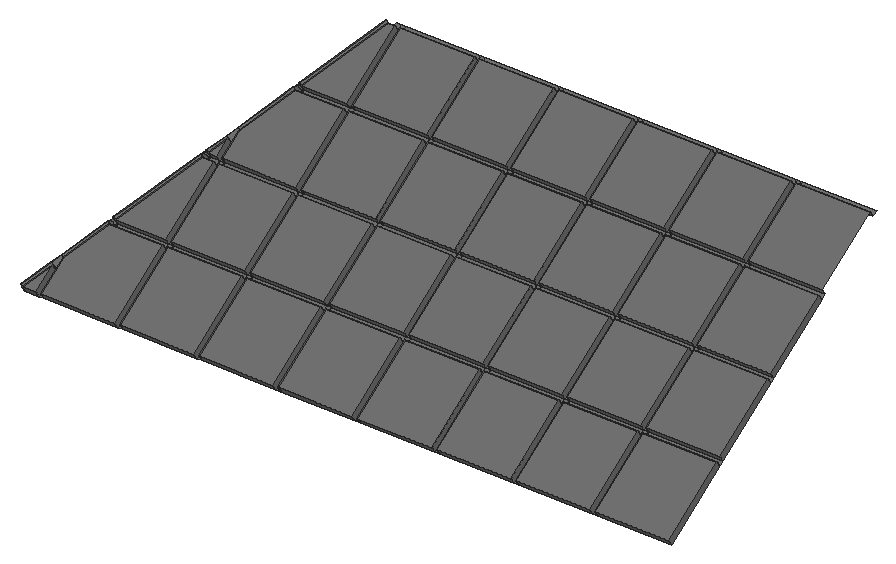
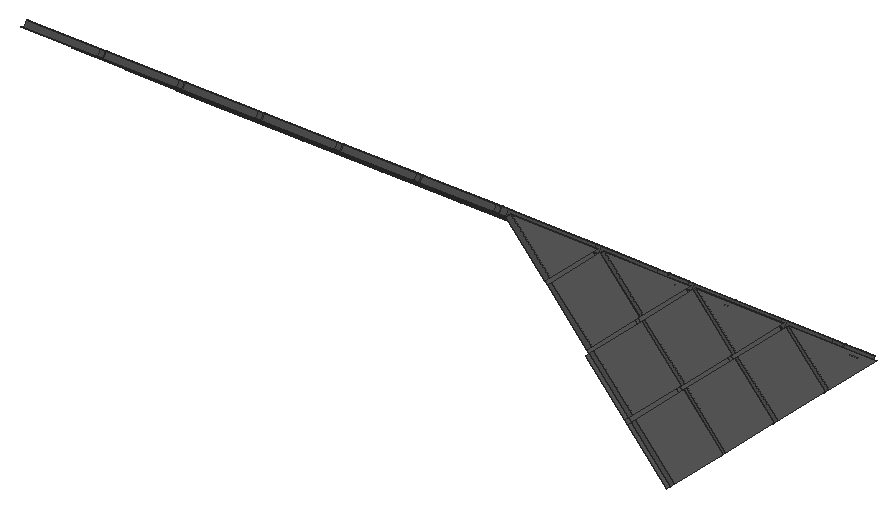
# SketchUp Ruby script. Lengths in inches.
U = 1.inch
M = Sketchup.active_model
def pt(a) = Geom::Point3d.new(a.map { |v| v * U })
def face(e, loops, mat)
  f = e.add_face(loops[0].map { |a| pt(a) })
  loops[1..].each { |l| e.add_face(l.map { |a| pt(a) }).erase! }
  f.material = f.back_material = mat if mat
  f
end
# faces: each face lists its corners as indices into pts; further lists are holes
def faces(e, pts, list, mat = nil) = list.each { |f| face(e, (f[0].is_a?(Array) ? f : [f]).map { |l| l.map { |i| pts[i] } }, mat) }
# xy, xz, yz: faces in a plane at the given z, y or x. An outline is a flat list of corners, or four numbers for a rectangle; further outlines are holes
def ring(l) = l.size == 4 ? [[l[0], l[1]], [l[2], l[1]], [l[2], l[3]], [l[0], l[3]]] : l.each_slice(2).to_a
def flat(e, list, mat, &to3) = list.each { |f| face(e, (f[0].is_a?(Array) ? f : [f]).map { |l| ring(l).map { |u, v| to3.(u, v) } }, mat) }
def xy(e, z, list, mat = nil) = flat(e, list, mat) { |x, y| [x, y, z] }
def xz(e, y, list, mat = nil) = flat(e, list, mat) { |x, z| [x, y, z] }
def yz(e, x, list, mat = nil) = flat(e, list, mat) { |y, z| [x, y, z] }
def lines(e, pts, list) = list.each { |a, b| e.add_line(pt(pts[a]), pt(pts[b])) }
# prism: a flat outline (further loops are holes) pulled along v
def prism(e, loops, v, mat = nil)
  f = face(e, loops, mat); d = Geom::Vector3d.new(v.map { |x| x * U })
  f.pushpull(f.normal.samedirection?(d) ? d.length : -d.length)
end
def box(e, o, s, mat = nil) = prism(e, [[o, [o[0] + s[0], o[1], o[2]], [o[0] + s[0], o[1] + s[1], o[2]], [o[0], o[1] + s[1], o[2]]]], [0, 0, s[2]], mat)
def at(x, y, z, deg = 0) = Geom::Transformation.translation(pt([x, y, z])) * Geom::Transformation.rotation(ORIGIN, Z_AXIS, deg.degrees)
def axes(o, x, y, z) = Geom::Transformation.new([*x, 0, *y, 0, *z, 0, *pt(o).to_a, 1])
def part(name) = M.definitions.add(name)
# library, detail: a bought-in or finely detailed component or shape, given as its bounding box
def library(name, o, s) = part(name).tap { |d| box(d.entities, o, s) }
def detail(e, o, s) = box(e.add_group.entities, o, s)
def put(e, d, t, mat = nil) = e.add_instance(d, t).tap { |i| i.material = mat if mat }
def group(e, t, mat = nil) = e.add_group.tap { |g| g.transformation = t; g.material = mat if mat }.entities
root = M.entities
M.materials.add("[Color M05]").color = [114, 114, 114]
xz(root,356.11,[[371.99,444.64,370.5,445.97,382.4,459.26,383.89,457.92]],"[Color M05]")
xz(root,357.32,[[371.99,444.64,383.89,457.92,382.4,459.26,370.5,445.97]],"[Color M05]")
xz(root,375.48,[[371.99,444.64,370.5,445.97,382.4,459.26,383.89,457.92],[384.68,458.81,383.1875,460.14,395.08,473.43,396.57,472.1]],"[Color M05]")
xz(root,376.69,[[371.99,444.64,383.89,457.92,382.4,459.26,370.5,445.97],[384.68,458.81,396.57,472.1,395.08,473.43,383.1875,460.14]],"[Color M05]")
xz(root,394.85,[[371.99,444.64,370.5,445.97,382.4,459.26,383.89,457.92],[384.68,458.81,383.1875,460.14,395.08,473.43,396.57,472.1],[397.37,472.98,395.88,474.32,407.77,487.6,409.26,486.27]],"[Color M05]")
xz(root,396.0625,[[371.99,444.64,383.89,457.92,382.4,459.26,370.5,445.97],[384.68,458.81,396.57,472.1,395.08,473.43,383.1875,460.14],[397.37,472.98,409.26,486.27,407.77,487.6,395.88,474.32]],"[Color M05]")
xz(root,414.22,[[371.99,444.64,370.5,445.97,382.4,459.26,383.89,457.92],[384.68,458.81,383.1875,460.14,395.08,473.43,396.57,472.1],[397.37,472.98,395.88,474.32,407.77,487.6,409.26,486.27],[410.06,487.15,408.57,488.49,420.46,501.77,421.95,500.4375]],"[Color M05]")
yz(root,376.12,[[337.95,444.64,344.26,449.25,343.08,450.87,336.77,446.25]],"[Color M05]")
yz(root,377.62,[[337.95,444.64,336.77,446.25,345.37,452.54,346.55,450.93]],"[Color M05]")
yz(root,400.12,[[337.95,444.64,356.11,457.92,354.93,459.54,336.77,446.25],[357.32,458.81,375.48,472.1,374.3,473.71,356.14,460.42],[376.69,472.98,380.9,476.06,379.72,477.67,375.51,474.6]],"[Color M05]")
yz(root,401.62,[[337.95,444.64,336.77,446.25,354.93,459.54,356.11,457.92],[357.32,458.81,356.14,460.42,374.3,473.71,375.48,472.1],[376.69,472.98,375.51,474.6,382.01,479.35,383.1875,477.73]],"[Color M05]")
yz(root,424.12,[[337.95,444.64,356.11,457.92,354.93,459.54,336.77,446.25],[357.32,458.81,375.48,472.1,374.3,473.71,356.14,460.42],[376.69,472.98,394.85,486.27,393.67,487.88,375.51,474.6],[396.0625,487.15,414.22,500.4375,413.04,502.05,394.88,488.77]],"[Color M05]")
yz(root,425.62,[[337.95,444.64,336.77,446.25,354.93,459.54,356.11,457.92],[357.32,458.81,356.14,460.42,374.3,473.71,375.48,472.1],[376.69,472.98,375.51,474.6,393.67,487.88,394.85,486.27],[396.0625,487.15,394.88,488.77,413.04,502.05,414.22,500.4375]],"[Color M05]")
yz(root,448.12,[[337.95,444.64,356.11,457.92,354.93,459.54,336.77,446.25],[357.32,458.81,375.48,472.1,374.3,473.71,356.14,460.42],[376.69,472.98,394.85,486.27,393.67,487.88,375.51,474.6],[396.0625,487.15,414.22,500.4375,413.04,502.05,394.88,488.77]],"[Color M05]")
yz(root,449.62,[[337.95,444.64,336.77,446.25,354.93,459.54,356.11,457.92],[357.32,458.81,356.14,460.42,374.3,473.71,375.48,472.1],[376.69,472.98,375.51,474.6,393.67,487.88,394.85,486.27],[396.0625,487.15,394.88,488.77,413.04,502.05,414.22,500.4375]],"[Color M05]")
yz(root,472.12,[[337.95,444.64,356.11,457.92,354.93,459.54,336.77,446.25],[357.32,458.81,375.48,472.1,374.3,473.71,356.14,460.42],[376.69,472.98,394.85,486.27,393.67,487.88,375.51,474.6],[396.0625,487.15,414.22,500.4375,413.04,502.05,394.88,488.77]],"[Color M05]")
yz(root,473.62,[[337.95,444.64,336.77,446.25,354.93,459.54,356.11,457.92],[357.32,458.81,356.14,460.42,374.3,473.71,375.48,472.1],[376.69,472.98,375.51,474.6,393.67,487.88,394.85,486.27],[396.0625,487.15,394.88,488.77,413.04,502.05,414.22,500.4375]],"[Color M05]")
yz(root,496.12,[[337.95,444.64,356.11,457.92,354.93,459.54,336.77,446.25],[357.32,458.81,375.48,472.1,374.3,473.71,356.14,460.42],[376.69,472.98,394.85,486.27,393.67,487.88,375.51,474.6],[396.0625,487.15,414.22,500.4375,413.04,502.05,394.88,488.77]],"[Color M05]")
yz(root,497.62,[[337.95,444.64,336.77,446.25,354.93,459.54,356.11,457.92],[357.32,458.81,356.14,460.42,374.3,473.71,375.48,472.1],[376.69,472.98,375.51,474.6,393.67,487.88,394.85,486.27],[396.0625,487.15,394.88,488.77,413.04,502.05,414.22,500.4375]],"[Color M05]")
yz(root,520.12,[[337.95,444.64,356.11,457.92,354.93,459.54,336.77,446.25],[357.32,458.81,375.48,472.1,374.3,473.71,356.14,460.42],[376.69,472.98,394.85,486.27,393.67,487.88,375.51,474.6],[396.0625,487.15,414.22,500.4375,413.04,502.05,394.88,488.77]],"[Color M05]")
yz(root,521.62,[[337.95,444.64,336.77,446.25,354.93,459.54,356.11,457.92],[357.32,458.81,356.14,460.42,374.3,473.71,375.48,472.1],[376.69,472.98,375.51,474.6,393.67,487.88,394.85,486.27],[396.0625,487.15,394.88,488.77,413.04,502.05,414.22,500.4375]],"[Color M05]")
yz(root,544.12,[[337.95,444.64,356.11,457.92,354.93,459.54,336.77,446.25],[357.32,458.81,375.48,472.1,374.3,473.71,356.14,460.42],[376.69,472.98,394.85,486.27,393.67,487.88,375.51,474.6],[396.0625,487.15,414.22,500.4375,413.04,502.05,394.88,488.77]],"[Color M05]")
yz(root,545.62,[[337.95,444.64,336.77,446.25,354.93,459.54,356.11,457.92],[357.32,458.81,356.14,460.42,374.3,473.71,375.48,472.1],[376.69,472.98,375.51,474.6,393.67,487.88,394.85,486.27],[396.0625,487.15,394.88,488.77,413.04,502.05,414.22,500.4375]],"[Color M05]")
yz(root,568.12,[[337.95,444.64,356.11,457.92,354.93,459.54,336.77,446.25],[357.32,458.81,375.48,472.1,374.3,473.71,356.14,460.42],[376.69,472.98,394.85,486.27,393.67,487.88,375.51,474.6]],"[Color M05]")
p = [[371.99,337.95,444.64],[376.12,337.95,444.64],[376.12,336.77,446.25],[371.99,336.77,446.25],[376.12,344.26,449.25],[376.12,343.08,450.87],
  [377.62,337.95,444.64],[400.12,337.95,444.64],[400.12,336.77,446.25],[377.62,336.77,446.25],[401.62,337.95,444.64],[424.12,337.95,444.64],
  [424.12,336.77,446.25],[401.62,336.77,446.25],[425.62,337.95,444.64],[448.12,337.95,444.64],[448.12,336.77,446.25],[425.62,336.77,446.25],
  [449.62,337.95,444.64],[472.12,337.95,444.64],[472.12,336.77,446.25],[449.62,336.77,446.25],[473.62,337.95,444.64],[496.12,337.95,444.64],
  [496.12,336.77,446.25],[473.62,336.77,446.25],[497.62,337.95,444.64],[520.12,337.95,444.64],[520.12,336.77,446.25],[497.62,336.77,446.25],
  [521.62,337.95,444.64],[544.12,337.95,444.64],[544.12,336.77,446.25],[521.62,336.77,446.25],[545.62,337.95,444.64],[568.12,337.95,444.64],
  [568.12,336.77,446.25],[545.62,336.77,446.25],[374.63,344.26,450.59],[370.5,337.95,445.97],[371.99,356.11,444.64],[370.5,356.11,445.97],
  [377.62,346.55,450.93],[401.62,356.11,457.92],[400.12,356.11,457.92],[425.62,356.11,457.92],[424.12,356.11,457.92],[449.62,356.11,457.92],
  [448.12,356.11,457.92],[473.62,356.11,457.92],[472.12,356.11,457.92],[497.62,356.11,457.92],[496.12,356.11,457.92],[521.62,356.11,457.92],
  [520.12,356.11,457.92],[545.62,356.11,457.92],[544.12,356.11,457.92],[371.99,357.32,444.64],[383.89,356.11,457.92],[383.89,357.32,457.92],
  [371.99,375.48,444.64],[370.5,357.32,445.97],[370.5,375.48,445.97],[383.89,375.48,457.92],[383.89,376.69,457.92],[371.99,376.69,444.64],
  [371.99,394.85,444.64],[370.5,376.69,445.97],[370.5,394.85,445.97],[371.99,396.0625,444.64],[383.89,394.85,457.92],[383.89,396.0625,457.92],
  [371.99,414.22,444.64],[370.5,396.0625,445.97],[370.5,414.22,445.97],[371.99,415.43,444.64],[383.89,414.22,457.92],[383.89,415.43,457.92],
  [376.13,346.55,452.26],[382.4,356.11,459.26],[382.4,357.32,459.26],[382.4,375.48,459.26],[382.4,376.69,459.26],[382.4,394.85,459.26],
  [382.4,396.0625,459.26],[382.4,414.22,459.26],[400.12,354.93,459.54],[383.89,354.93,459.54],[377.62,345.37,452.54],[424.12,354.93,459.54],
  [401.62,354.93,459.54],[448.12,354.93,459.54],[425.62,354.93,459.54],[472.12,354.93,459.54],[449.62,354.93,459.54],[496.12,354.93,459.54],
  [473.62,354.93,459.54],[520.12,354.93,459.54],[497.62,354.93,459.54],[544.12,354.93,459.54],[521.62,354.93,459.54],[568.12,354.93,459.54],
  [545.62,354.93,459.54],[568.12,356.11,457.92],[400.12,357.32,458.81],[384.68,357.32,458.81],[401.62,357.32,458.81],[424.12,357.32,458.81],
  [425.62,357.32,458.81],[448.12,357.32,458.81],[449.62,357.32,458.81],[472.12,357.32,458.81],[473.62,357.32,458.81],[496.12,357.32,458.81],
  [497.62,357.32,458.81],[520.12,357.32,458.81],[521.62,357.32,458.81],[544.12,357.32,458.81],[545.62,357.32,458.81],[568.12,357.32,458.81],
  [384.68,375.48,458.81],[384.68,376.69,458.81],[384.68,394.85,458.81],[384.68,396.0625,458.81],[384.68,414.22,458.81],[384.68,415.43,458.81],
  [400.12,356.14,460.42],[384.68,356.14,460.42],[396.57,375.48,472.1],[396.57,374.3,473.71],[424.12,356.14,460.42],[401.62,356.14,460.42],
  [448.12,356.14,460.42],[425.62,356.14,460.42],[472.12,356.14,460.42],[449.62,356.14,460.42],[496.12,356.14,460.42],[473.62,356.14,460.42],
  [520.12,356.14,460.42],[497.62,356.14,460.42],[544.12,356.14,460.42],[521.62,356.14,460.42],[568.12,356.14,460.42],[545.62,356.14,460.42],
  [383.1875,357.32,460.14],[383.1875,375.48,460.14],[395.08,375.48,473.43],[401.62,375.48,472.1],[400.12,375.48,472.1],[425.62,375.48,472.1],
  [424.12,375.48,472.1],[449.62,375.48,472.1],[448.12,375.48,472.1],[473.62,375.48,472.1],[472.12,375.48,472.1],[497.62,375.48,472.1],
  [496.12,375.48,472.1],[521.62,375.48,472.1],[520.12,375.48,472.1],[545.62,375.48,472.1],[544.12,375.48,472.1],[396.57,376.69,472.1],
  [383.1875,376.69,460.14],[383.1875,394.85,460.14],[396.57,394.85,472.1],[396.57,396.0625,472.1],[383.1875,396.0625,460.14],[383.1875,414.22,460.14],
  [396.57,414.22,472.1],[396.57,415.43,472.1],[395.08,376.69,473.43],[395.08,394.85,473.43],[395.08,396.0625,473.43],[395.08,414.22,473.43],
  [400.12,374.3,473.71],[424.12,374.3,473.71],[401.62,374.3,473.71],[448.12,374.3,473.71],[425.62,374.3,473.71],[472.12,374.3,473.71],
  [449.62,374.3,473.71],[496.12,374.3,473.71],[473.62,374.3,473.71],[520.12,374.3,473.71],[497.62,374.3,473.71],[544.12,374.3,473.71],
  [521.62,374.3,473.71],[568.12,374.3,473.71],[545.62,374.3,473.71],[568.12,375.48,472.1],[400.12,376.69,472.98],[397.37,376.69,472.98],
  [401.62,376.69,472.98],[424.12,376.69,472.98],[425.62,376.69,472.98],[448.12,376.69,472.98],[449.62,376.69,472.98],[472.12,376.69,472.98],
  [473.62,376.69,472.98],[496.12,376.69,472.98],[497.62,376.69,472.98],[520.12,376.69,472.98],[521.62,376.69,472.98],[544.12,376.69,472.98],
  [545.62,376.69,472.98],[568.12,376.69,472.98],[397.37,394.85,472.98],[397.37,396.0625,472.98],[397.37,414.22,472.98],[400.12,375.51,474.6],
  [397.37,375.51,474.6],[400.12,380.9,476.06],[400.12,379.72,477.67],[424.12,375.51,474.6],[401.62,375.51,474.6],[448.12,375.51,474.6],
  [425.62,375.51,474.6],[472.12,375.51,474.6],[449.62,375.51,474.6],[496.12,375.51,474.6],[473.62,375.51,474.6],[520.12,375.51,474.6],
  [497.62,375.51,474.6],[544.12,375.51,474.6],[521.62,375.51,474.6],[568.12,375.51,474.6],[545.62,375.51,474.6],[398.63,380.9,477.39],
  [395.88,376.69,474.32],[395.88,394.85,474.32],[401.62,383.1875,477.73],[425.62,394.85,486.27],[424.12,394.85,486.27],[449.62,394.85,486.27],
  [448.12,394.85,486.27],[473.62,394.85,486.27],[472.12,394.85,486.27],[497.62,394.85,486.27],[496.12,394.85,486.27],[521.62,394.85,486.27],
  [520.12,394.85,486.27],[545.62,394.85,486.27],[544.12,394.85,486.27],[409.26,394.85,486.27],[409.26,396.0625,486.27],[395.88,396.0625,474.32],
  [395.88,414.22,474.32],[400.13,383.1875,479.07],[407.77,394.85,487.6],[407.77,396.0625,487.6],[407.77,414.22,487.6],[424.12,393.67,487.88],
  [409.26,393.67,487.88],[401.62,382.01,479.35],[448.12,393.67,487.88],[425.62,393.67,487.88],[472.12,393.67,487.88],[449.62,393.67,487.88],
  [496.12,393.67,487.88],[473.62,393.67,487.88],[520.12,393.67,487.88],[497.62,393.67,487.88],[544.12,393.67,487.88],[521.62,393.67,487.88],
  [568.12,393.67,487.88],[545.62,393.67,487.88],[568.12,394.85,486.27],[424.12,396.0625,487.15],[410.06,396.0625,487.15],[425.62,396.0625,487.15],
  [448.12,396.0625,487.15],[449.62,396.0625,487.15],[472.12,396.0625,487.15],[473.62,396.0625,487.15],[496.12,396.0625,487.15],[497.62,396.0625,487.15],
  [520.12,396.0625,487.15],[521.62,396.0625,487.15],[544.12,396.0625,487.15],[545.62,396.0625,487.15],[568.12,396.0625,487.15],[409.26,414.22,486.27],
  [410.06,414.22,487.15],[424.12,394.88,488.77],[410.06,394.88,488.77],[421.95,414.22,500.4375],[421.95,413.04,502.05],[448.12,394.88,488.77],
  [425.62,394.88,488.77],[472.12,394.88,488.77],[449.62,394.88,488.77],[496.12,394.88,488.77],[473.62,394.88,488.77],[520.12,394.88,488.77],
  [497.62,394.88,488.77],[544.12,394.88,488.77],[521.62,394.88,488.77],[568.12,394.88,488.77],[545.62,394.88,488.77],[408.57,396.0625,488.49],
  [408.57,414.22,488.49],[420.46,414.22,501.77],[425.62,414.22,500.4375],[424.12,414.22,500.4375],[449.62,414.22,500.4375],[448.12,414.22,500.4375],
  [473.62,414.22,500.4375],[472.12,414.22,500.4375],[497.62,414.22,500.4375],[496.12,414.22,500.4375],[521.62,414.22,500.4375],[520.12,414.22,500.4375],
  [545.62,414.22,500.4375],[544.12,414.22,500.4375],[424.12,413.04,502.05],[448.12,413.04,502.05],[425.62,413.04,502.05],[472.12,413.04,502.05],
  [449.62,413.04,502.05],[496.12,413.04,502.05],[473.62,413.04,502.05],[520.12,413.04,502.05],[497.62,413.04,502.05],[544.12,413.04,502.05],
  [521.62,413.04,502.05],[568.12,413.04,502.05],[545.62,413.04,502.05],[568.12,414.22,500.4375],[424.12,415.43,501.32],[422.75,415.43,501.32],
  [425.62,415.43,501.32],[448.12,415.43,501.32],[449.62,415.43,501.32],[472.12,415.43,501.32],[473.62,415.43,501.32],[496.12,415.43,501.32],
  [497.62,415.43,501.32],[520.12,415.43,501.32],[521.62,415.43,501.32],[544.12,415.43,501.32],[545.62,415.43,501.32],[568.12,415.43,501.32]]
faces(root,p,[[0,1,2,3],[4,0,3,5],[6,7,8,9],[10,11,12,13],[14,15,16,17],[18,19,20,21],[22,23,24,25],[26,27,28,29],
  [30,31,32,33],[34,35,36,37],[0,4,38,39],[40,0,39,41],[1,6,42,4],[7,10,43,44],[11,14,45,46],[15,18,47,48],
  [19,22,49,50],[23,26,51,52],[27,30,53,54],[31,34,55,56],[57,40,58,59],[60,57,61,62],[63,64,65,60],[66,65,67,68],
  [69,66,70,71],[72,69,73,74],[75,72,76,77],[78,79,41,39,38],[62,61,80,81],[68,67,82,83],[74,73,84,85],[3,2,5],
  [9,8,86,87,88],[13,12,89,90],[17,16,91,92],[21,20,93,94],[25,24,95,96],[29,28,97,98],[33,32,99,100],[37,36,101,102],
  [4,42,78,38],[58,42,88,87],[42,58,79,78],[44,58,87,86],[46,43,90,89],[48,45,92,91],[50,47,94,93],[52,49,96,95],
  [54,51,98,97],[56,53,100,99],[103,55,102,101],[58,44,104,105],[58,105,59],[44,43,106,104],[43,46,107,106],[46,45,108,107],
  [45,48,109,108],[48,47,110,109],[47,50,111,110],[50,49,112,111],[49,52,113,112],[52,51,114,113],[51,54,115,114],[54,53,116,115],
  [53,56,117,116],[56,55,118,117],[55,103,119,118],[59,63,81,80],[63,59,105,120],[120,121,64,63],[64,70,83,82],[70,64,121,122],
  [71,70,122,123],[71,76,85,84],[76,71,123,124],[77,76,124,125],[105,104,126,127],[128,105,127,129],[106,107,130,131],[108,109,132,133],
  [110,111,134,135],[112,113,136,137],[114,115,138,139],[116,117,140,141],[118,119,142,143],[120,105,144,145],[105,128,146,144],[104,106,147,148],
  [107,108,149,150],[109,110,151,152],[111,112,153,154],[113,114,155,156],[115,116,157,158],[117,118,159,160],[128,161,121,120],[122,121,162,163],
  [123,122,164,165],[124,123,166,167],[125,124,168,169],[144,146,145],[163,162,170,171],[167,166,172,173],[127,126,174,129],[131,130,175,176],
  [133,132,177,178],[135,134,179,180],[137,136,181,182],[139,138,183,184],[141,140,185,186],[143,142,187,188],[148,128,129,174],[150,147,176,175],
  [152,149,178,177],[154,151,180,179],[156,153,182,181],[158,155,184,183],[160,157,186,185],[189,159,188,187],[128,148,190,191],[128,191,161],
  [148,147,192,190],[147,150,193,192],[150,149,194,193],[149,152,195,194],[152,151,196,195],[151,154,197,196],[154,153,198,197],[153,156,199,198],
  [156,155,200,199],[155,158,201,200],[158,157,202,201],[157,160,203,202],[160,159,204,203],[159,189,205,204],[161,164,171,170],[164,161,191,206],
  [165,164,206,207],[165,168,173,172],[168,165,207,208],[191,190,209,210],[211,191,210,212],[192,193,213,214],[194,195,215,216],[196,197,217,218],
  [198,199,219,220],[200,201,221,222],[202,203,223,224],[204,205,225,226],[191,211,227,228],[206,191,228,229],[190,192,230,211],[193,194,231,232],
  [195,196,233,234],[197,198,235,236],[199,200,237,238],[201,202,239,240],[203,204,241,242],[207,206,243,244],[208,207,245,246],[247,248,229,228,227],
  [246,245,249,250],[210,209,212],[214,213,251,252,253],[216,215,254,255],[218,217,256,257],[220,219,258,259],[222,221,260,261],[224,223,262,263],
  [226,225,264,265],[211,230,247,227],[243,230,253,252],[230,243,248,247],[232,243,252,251],[234,231,255,254],[236,233,257,256],[238,235,259,258],
  [240,237,261,260],[242,239,263,262],[266,241,265,264],[243,232,267,268],[243,268,244],[232,231,269,267],[231,234,270,269],[234,233,271,270],
  [233,236,272,271],[236,235,273,272],[235,238,274,273],[238,237,275,274],[237,240,276,275],[240,239,277,276],[239,242,278,277],[242,241,279,278],
  [241,266,280,279],[244,281,250,249],[281,244,268,282],[268,267,283,284],[285,268,284,286],[269,270,287,288],[271,272,289,290],[273,274,291,292],
  [275,276,293,294],[277,278,295,296],[279,280,297,298],[282,268,299,300],[268,285,301,299],[267,269,302,303],[270,271,304,305],[272,273,306,307],
  [274,275,308,309],[276,277,310,311],[278,279,312,313],[299,301,300],[284,283,314,286],[288,287,315,316],[290,289,317,318],[292,291,319,320],
  [294,293,321,322],[296,295,323,324],[298,297,325,326],[303,285,286,314],[305,302,316,315],[307,304,318,317],[309,306,320,319],[311,308,322,321],
  [313,310,324,323],[327,312,326,325],[285,303,328,329],[303,302,330,328],[302,305,331,330],[305,304,332,331],[304,307,333,332],[307,306,334,333],
  [306,309,335,334],[309,308,336,335],[308,311,337,336],[311,310,338,337],[310,313,339,338],[313,312,340,339],[312,327,341,340]],"[Color M05]")
